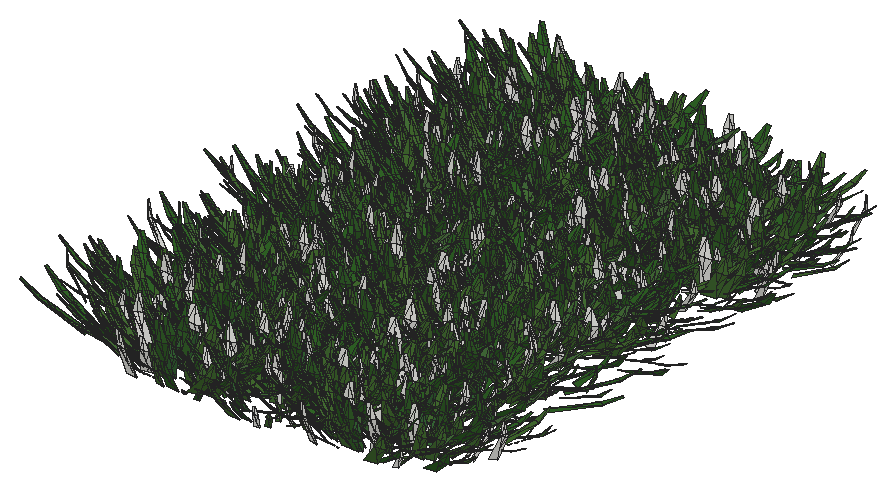
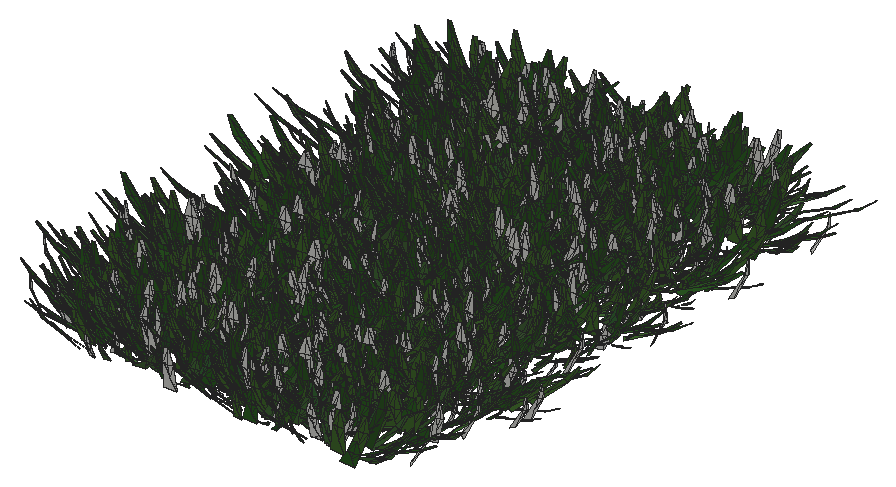
# SketchUp Ruby script. Lengths in inches.
U = 1.inch
M = Sketchup.active_model
def pt(a) = Geom::Point3d.new(a.map { |v| v * U })
def face(e, loops, mat)
  f = e.add_face(loops[0].map { |a| pt(a) })
  loops[1..].each { |l| e.add_face(l.map { |a| pt(a) }).erase! }
  f.material = f.back_material = mat if mat
  f
end
# faces: each face lists its corners as indices into pts; further lists are holes
def faces(e, pts, list, mat = nil) = list.each { |f| face(e, (f[0].is_a?(Array) ? f : [f]).map { |l| l.map { |i| pts[i] } }, mat) }
# xy, xz, yz: faces in a plane at the given z, y or x. An outline is a flat list of corners, or four numbers for a rectangle; further outlines are holes
def ring(l) = l.size == 4 ? [[l[0], l[1]], [l[2], l[1]], [l[2], l[3]], [l[0], l[3]]] : l.each_slice(2).to_a
def flat(e, list, mat, &to3) = list.each { |f| face(e, (f[0].is_a?(Array) ? f : [f]).map { |l| ring(l).map { |u, v| to3.(u, v) } }, mat) }
def xy(e, z, list, mat = nil) = flat(e, list, mat) { |x, y| [x, y, z] }
def xz(e, y, list, mat = nil) = flat(e, list, mat) { |x, z| [x, y, z] }
def yz(e, x, list, mat = nil) = flat(e, list, mat) { |y, z| [x, y, z] }
def lines(e, pts, list) = list.each { |a, b| e.add_line(pt(pts[a]), pt(pts[b])) }
# prism: a flat outline (further loops are holes) pulled along v
def prism(e, loops, v, mat = nil)
  f = face(e, loops, mat); d = Geom::Vector3d.new(v.map { |x| x * U })
  f.pushpull(f.normal.samedirection?(d) ? d.length : -d.length)
end
def box(e, o, s, mat = nil) = prism(e, [[o, [o[0] + s[0], o[1], o[2]], [o[0] + s[0], o[1] + s[1], o[2]], [o[0], o[1] + s[1], o[2]]]], [0, 0, s[2]], mat)
def at(x, y, z, deg = 0) = Geom::Transformation.translation(pt([x, y, z])) * Geom::Transformation.rotation(ORIGIN, Z_AXIS, deg.degrees)
def axes(o, x, y, z) = Geom::Transformation.new([*x, 0, *y, 0, *z, 0, *pt(o).to_a, 1])
def part(name) = M.definitions.add(name)
# library, detail: a bought-in or finely detailed component or shape, given as its bounding box
def library(name, o, s) = part(name).tap { |d| box(d.entities, o, s) }
def detail(e, o, s) = box(e.add_group.entities, o, s)
def put(e, d, t, mat = nil) = e.add_instance(d, t).tap { |i| i.material = mat if mat }
def group(e, t, mat = nil) = e.add_group.tap { |g| g.transformation = t; g.material = mat if mat }.entities
root = M.entities
M.materials.add("Material82").color = [68, 110, 58]
M.materials.add("Material83").color = [48, 90, 38]
M.materials.add("Material84").color = [68, 110, 48]
M.materials.add("Material85").color = [48, 90, 48]
M.materials.add("Material86").color = [58, 110, 58]
M.materials.add("Material87").color = [58, 90, 38]
M.materials.add("Material88").color = [68, 100, 58]
M.materials.add("Material89").color = [48, 100, 38]
c1 = part("grass00")
p = [[-0.6875,0.15,0],[-0.56,0.08,5.52],[-0.04,0.03,2.76],[0.48,-0.02,0],[0.35,-0.02,5.52],[-0.1,-0.14,5.52],
  [-0.12,0.65,8.37],[-0.42,0.65,8.37]]
faces(c1.entities,p,[[0,1,2,3],[3,2,4],[1,5,2],[5,4,2],[1,6,5],[4,5,6],[7,6,1]])
c2 = part("Group16\#1")
put(c2.entities,c1,axes([1.44,-0.61,-0.01],[0.05352,0.12609,0],[-0.10704,0.04543,0.07239],[0.06664,-0.02828,0.11628]),"Material85")
put(c2.entities,c1,axes([0.76,-0.15,-0.01],[0.04676,0.24062,0],[-0.23162,0.04501,0.06642],[0.0652,-0.01267,0.23595]),"Material82")
put(c2.entities,c1,axes([0.79,0.01,-0.01],[-0.00606,0.34651,0],[-0.34381,-0.00602,0.0432],[0.04319,0.00076,0.34386]))
put(c2.entities,c1,axes([1,0.23,-0.01],[-0.07192,0.31144,0],[-0.28722,-0.06632,0.1236],[0.12043,0.02781,0.29478]),"Material84")
put(c2.entities,c1,axes([1.66,0.77,-0.01],[-0.13828,0.29651,0],[-0.21551,-0.1005,0.22471],[0.20365,0.09498,0.23779]),"Material89")
put(c2.entities,c1,axes([0.6875,0.52,-0.01],[-0.18126,0.24051,0],[-0.22746,-0.17142,0.09788],[0.07817,0.05891,0.28481]),"Material84")
put(c2.entities,c1,axes([0.68,0.78,-0.01],[-0.215,0.18688,0],[-0.12385,-0.14248,0.21334],[0.13995,0.16101,0.18878]),"Material82")
put(c2.entities,c1,axes([0.56,1,-0.01],[-0.13756,0.07624,0],[-0.06159,-0.11112,0.0927],[0.04494,0.08108,0.12705]),"Material84")
put(c2.entities,c1,axes([0.2,0.64,-0.01],[-0.23729,0.07254,0],[-0.05711,-0.18681,0.153],[0.04473,0.14632,0.19535]),"Material89")
put(c2.entities,c1,axes([0.0625,0.72,-0.01],[-0.28874,0.02525,0],[-0.02179,-0.24916,0.14647],[0.01276,0.14591,0.25012]),"Material82")
put(c2.entities,c1,axes([-0.08,0.62,-0.01],[-0.34089,-0.04187,0],[0.03255,-0.26504,0.216],[-0.02633,0.21439,0.26703]),"Material89")
put(c2.entities,c1,axes([-0.34,0.98,-0.01],[-0.14314,-0.0493,0],[0.04397,-0.12769,0.06843],[-0.02228,0.0647,0.13505]),"Material89")
put(c2.entities,c1,axes([-0.87,1.45,-0.01],[-0.23488,-0.14114,0],[0.13761,-0.22901,0.06087],[-0.03135,0.05217,0.26717]))
put(c2.entities,c1,axes([-0.72,0.77,-0.01],[-0.14208,-0.13251,0],[0.07209,-0.0773,0.16301],[-0.11118,0.11922,0.1057]),"Material89")
put(c2.entities,c1,axes([-0.62,0.43,-0.01],[-0.14845,-0.21203,0],[0.18654,-0.13061,0.12304],[-0.10079,0.07057,0.22772]),"Material82")
put(c2.entities,c1,axes([-0.68,0.29,-0.01],[-0.13639,-0.32136,0],[0.31723,-0.13464,0.05579],[-0.05136,0.0218,0.34462]),"Material83")
put(c2.entities,c1,axes([-0.64,0.125,-0.01],[-0.0458,-0.23569,0],[0.22124,-0.043,0.08276],[-0.08124,0.01579,0.22538]),"Material86")
put(c2.entities,c1,axes([-1.6,-0.03,-0.01],[0.00576,-0.32897,0],[0.27526,0.00482,0.18018],[-0.18015,-0.00315,0.2753]),"Material84")
put(c2.entities,c1,axes([-1.36,-0.31,-0.01],[0.05718,-0.24765,0],[0.18172,0.04196,0.17267],[-0.16825,-0.03885,0.1865]),"Material89")
put(c2.entities,c1,axes([-1.54,-0.72,-0.01],[0.06537,-0.14017,0],[0.13555,0.06321,0.03939],[-0.0357,-0.01665,0.14956]))
put(c2.entities,c1,axes([-1.19,-0.9,-0.01],[0.09597,-0.12735,0],[0.11214,0.08451,0.07557],[-0.06035,-0.04548,0.14042]),"Material88")
put(c2.entities,c1,axes([-0.47,-0.54,-0.01],[0.11588,-0.10072,0],[0.0618,0.0711,0.12124],[-0.07953,-0.0915,0.0942]))
put(c2.entities,c1,axes([-0.47,-0.84,-0.01],[0.11927,-0.0661,0],[0.06603,0.11913,0.00646],[-0.00313,-0.00565,0.13621]),"Material84")
put(c2.entities,c1,axes([-0.38,-1.24,-0.01],[0.28037,-0.08571,0],[0.0618,0.20215,0.20315],[-0.05939,-0.19428,0.21139]),"Material88")
put(c2.entities,c1,axes([-0.06,-0.66,-0.01],[0.22719,-0.01987,0],[0.01247,0.14255,0.17758],[-0.01547,-0.17691,0.1431]),"Material87")
put(c2.entities,c1,axes([0.11,-0.89,-0.01],[0.14882,0.01828,0],[-0.01058,0.08611,0.12229],[0.01491,-0.12138,0.08676]),"Material85")
put(c2.entities,c1,axes([0.25,-0.72,-0.01],[0.20481,0.07053,0],[-0.06206,0.18022,0.10291],[0.03351,-0.0973,0.1906]),"Material85")
put(c2.entities,c1,axes([0.85,-1.42,-0.01],[0.16481,0.09904,0],[-0.09472,0.15762,0.05616],[0.02893,-0.04814,0.18389]),"Material84")
put(c2.entities,c1,axes([1.01,-1.09,-0.01],[0.21858,0.20385,0],[-0.17495,0.1876,0.15339],[0.10462,-0.11218,0.25652]),"Material89")
put(c2.entities,c1,axes([1.01,-0.71,-0.01],[0.08733,0.12473,0],[-0.06445,0.04512,0.13037],[0.1068,-0.07477,0.07867]),"Material85")
c3 = part("Group15\#1")
put(c3.entities,c2,at(0,0,0))
c4 = part("3darcstudiotree_grass00\#1")
put(c4.entities,c3,at(0,0,0))
put(root,c4,axes([1794.49,955.9,-29.74],[2.02269,1.40625,0],[-2.88305,0.64496,-0.03898],[-0.27125,0.06068,1.98748]))
put(root,c4,axes([1794.85,983.84,-29.74],[2.29641,1.07421,0],[-2.57105,0.85483,-0.04117],[-0.19383,0.06444,1.55213]))
put(root,c4,axes([1794.83,946.6,-29.74],[0.20899,1.64265,0],[-4.27343,0.08456,-0.03261],[-0.1888,0.00374,1.85888]))
put(root,c4,axes([1794.68,966.71,-29.74],[1.08869,1.44245,0],[-3.40274,0.39943,-0.00785],[-0.05372,0.00631,1.89978]))
put(root,c4,axes([1794.9,981.94,-29.74],[2.7006,1.1614,0],[-2.43909,0.8821,-0.03804],[-0.19893,0.07194,1.7602]))
put(root,c4,axes([1797.5625,973.19,-29.74],[-2.45174,-1.03973,0],[2.50397,-0.91832,-0.03633],[0.18002,-0.06602,1.73438]))
put(root,c4,axes([1797.66,970.78,-29.74],[-1.7758,-1.16797,0],[3.11451,-0.73649,-0.04451],[0.21848,-0.05166,1.55797]))
put(root,c4,axes([1798.16,960.11,-29.74],[-4.0045,-0.70324,0],[1.53901,-1.36302,-0.04343],[0.08424,-0.0746,1.35201]))
put(root,c4,axes([1797.9,953.62,-29.74],[-0.8562,-1.46222,0],[3.2715,-0.29793,-0.0292],[0.1741,-0.01586,1.53984]))
put(root,c4,axes([1797.63,961.45,-29.74],[2.12424,-1.58648,0],[2.98317,0.62124,-0.03491],[0.20173,0.04201,1.65255]))
put(root,c4,axes([1798.36,942.04,-29.74],[-3.45178,0.2701,0],[-0.90786,-1.80446,-0.05548],[-0.0508,-0.10098,1.6451]))
put(root,c4,axes([1799.49,982.04,-29.74],[-3.12186,-1.16816,0],[2.84193,-1.18123,-0.00166],[0.00643,-0.00267,1.74215]))
put(root,c4,axes([1797.65,988.83,-29.74],[3.25093,0.54248,0],[-1.41803,1.32165,-0.02719],[-0.07494,0.06985,1.929]))
put(root,c4,axes([1797.67,989.51,-29.74],[-0.25702,1.50589,0],[-4.4334,-0.11768,-0.01753],[-0.09867,-0.00262,1.87889]))
put(root,c4,axes([1797.58,967.875,-29.74],[3.97101,0.68213,0],[-1.55734,1.41002,-0.04191],[-0.07595,0.06876,1.32656]))
put(root,c4,axes([1798.15,995.21,-29.74],[0.4621,1.41992,0],[-4.03416,0.20419,-0.0516],[-0.33532,0.01697,1.99718]))
put(root,c4,axes([1797.97,977.52,-29.74],[4.12561,0.29265,0],[-0.72369,1.58676,-0.03729],[-0.0346,0.07587,1.60628]))
put(root,c4,axes([1799.72,950.6,-29.74],[-3.96689,-0.26306,0],[0.64548,-1.51387,-0.0114],[0.01279,-0.03,1.97478]))
put(root,c4,axes([1798.23,974.62,-29.74],[2.01819,1.66422,0],[-3.45385,0.65143,-0.02212],[-0.1358,0.02561,1.95299]))
put(root,c4,axes([1798.51,958.22,-29.74],[-0.26486,1.49696,0],[-3.89065,-0.10706,-0.02357],[-0.1242,-0.00342,1.54387]))
put(root,c4,axes([1798.52,948.51,-29.74],[4.24203,-0.02956,0],[0.08072,1.80172,-0.02875],[0.00231,0.05162,1.55972]))
put(root,c4,axes([1798.66,983.97,-29.74],[2.46344,0.86677,0],[-2.31784,1.02455,-0.00625],[-0.02756,0.01218,1.72796]))
put(root,c4,axes([1800.12,965.53,-29.74],[-3.7951,0.9119,0],[-2.12877,-1.37789,-0.05764],[-0.17628,-0.1141,1.8024]))
put(root,c4,axes([1800.5,944.45,-29.74],[1.13972,-1.41461,0],[4.50389,0.56436,-0.03698],[0.18209,0.02282,1.82987]))
put(root,c4,axes([1801.0625,954.77,-29.74],[-2.49551,-1.26471,0],[2.8619,-0.87828,-0.01663],[0.09126,-0.02801,1.89037]))
put(root,c4,axes([1800.7,940.35,-29.74],[-2.98133,1.10226,0],[-2.6348,-1.10837,-0.04557],[-0.21161,-0.08902,1.96028]))
put(root,c4,axes([1800.3125,978.84,-29.74],[-2.13819,1.22316,0],[-3.167,-0.86103,-0.02321],[-0.1127,-0.03064,1.70026]))
put(root,c4,axes([1800.97,947.39,-29.74],[-3.3677,0.38425,0],[-1.22656,-1.67195,-0.00573],[-0.0077,-0.0105,1.59925]))
put(root,c4,axes([1800.92,986.4,-29.74],[2.12809,-1.0558,0],[3.61722,1.13396,-0.06111],[0.24603,0.07713,1.78135]))
put(root,c4,axes([1801.03,993.1,-29.74],[3.47556,-0.63984,0],[1.81232,1.53108,-0.02938],[0.06383,0.05392,1.64954]))
put(root,c4,axes([1800.85,964.29,-29.74],[4.6709,-0.11713,0],[0.23839,1.47848,-0.03177],[0.01367,0.08477,1.90853]))
put(root,c4,axes([1803.0625,971.1,-29.74],[-3.65792,-0.8597,0],[1.995,-1.32021,-0.01663],[0.05672,-0.03754,1.94585]))
put(root,c4,axes([1803.21,940.4,-29.74],[3.22982,-1.36398,0],[2.52221,0.92889,-0.01281],[0.05669,0.02088,1.56626]))
put(root,c4,axes([1804.68,966.21,-29.74],[-1.61628,-1.19973,0],[3.67441,-0.7699,-0.00698],[0.03732,-0.00782,1.8873]))
put(root,c4,axes([1804.32,944.1875,-29.74],[1.53079,-1.5017,0],[4.19952,0.6658,-0.01772],[0.08663,0.01374,1.7874]))
put(root,c4,axes([1804.85,953.47,-29.74],[-3.12873,-1.31633,0],[2.88309,-1.0658,-0.03051],[0.12402,-0.04585,1.65027]))
put(root,c4,axes([1804.24,991.84,-29.74],[2.10607,-1.53284,0],[3.55653,0.76,-0.00988],[0.05409,0.01156,1.88737]))
put(root,c4,axes([1803.2,959.43,-29.74],[4.72899,0.01401,0],[-0.03317,1.74196,-0.012],[-0.00046,0.02441,1.70791]))
put(root,c4,axes([1803.95,942.24,-29.74],[3.14565,-0.76847,0],[1.85222,1.17921,-0.00486],[0.01386,0.00882,1.42853]))
put(root,c4,axes([1803.34,961.83,-29.74],[1.47307,1.52241,0],[-3.55442,0.5349,-0.03212],[-0.18221,0.02742,1.73128]))
put(root,c4,axes([1803.71,948.7,-29.74],[3.86384,0.07818,0],[-0.23972,1.84255,-0.05168],[-0.01275,0.09801,1.68853]))
put(root,c4,axes([1803.54,955.48,-29.74],[0.17144,1.84869,0],[-4.60552,0.06643,-0.0182],[-0.07619,0.0011,1.44668]))
put(root,c4,axes([1803.7,974.37,-29.74],[0.6087,1.43701,0],[-3.38203,0.22281,-0.00028],[-0.00164,0.00011,1.50491]))
put(root,c4,axes([1804.01,990.32,-29.74],[-0.11554,1.45354,0],[-4.02615,-0.04978,-0.04067],[-0.20655,-0.00255,1.53414]))
put(root,c4,axes([1804.83,981.89,-29.74],[-3.14808,1.22755,0],[-2.57668,-1.02773,-0.03762],[-0.14164,-0.05649,1.47105]))
put(root,c4,axes([1803.68,986.65,-29.74],[0.48824,1.58889,0],[-4.56618,0.21822,-0.01569],[-0.06712,0.00321,1.48562]))
put(root,c4,axes([1805.84,977.55,-29.74],[-3.3453,-1.30601,0],[3.28392,-1.30825,-0.03717],[0.14464,-0.05762,1.93537]))
put(root,c4,axes([1805.64,972.4,-29.74],[-4.03093,-0.26709,0],[0.61626,-1.44652,-0.01654],[0.01865,-0.04378,1.89711]))
put(root,c4,axes([1806.03,978.98,-29.74],[-1.63649,-1.29377,0],[3.38922,-0.66676,-0.00448],[0.02699,-0.00531,1.90991]))
put(root,c4,axes([1805.21,958.33,-29.74],[-3.19374,0.7238,0],[-2.32014,-1.59223,-0.04948],[-0.1132,-0.07768,1.60238]))
put(root,c4,axes([1804.66,984.03,-29.74],[0.67214,1.30105,0],[-3.68417,0.29602,-0.04728],[-0.27019,0.02171,1.64346]))
put(root,c4,axes([1804.99,968.28,-29.74],[3.23921,0.6316,0],[-1.61427,1.28761,-0.03066],[-0.08714,0.06951,1.75054]))
put(root,c4,axes([1806.09,947.34,-29.74],[0.38628,-1.42854,0],[3.50239,0.14729,-0.04937],[0.32013,0.01346,1.72169]))
put(root,c4,axes([1806.32,963.77,-29.74],[-1.61807,1.52118,0],[-3.6405,-0.60227,-0.04701],[-0.26943,-0.04457,1.83905]))
put(root,c4,axes([1806.52,951.08,-29.74],[0.41177,1.61489,0],[-3.5087,0.13914,-0.04963],[-0.27633,0.01096,1.47912]))
put(root,c4,axes([1805.89,994.14,-29.74],[3.03872,1.12896,0],[-3.11924,1.30579,-0.01047],[-0.04051,0.01696,1.92288]))
put(root,c4,axes([1806.92,987.59,-29.74],[3.86781,0.52244,0],[-1.13731,1.30954,-0.02009],[-0.0432,0.04974,1.7458]))
put(root,c4,axes([1808.63,986.48,-29.74],[-4.0386,-0.4374,0],[0.94795,-1.36128,-0.02848],[0.0516,-0.0741,1.83531]))
put(root,c4,axes([1808.37,992.54,-29.74],[-0.39879,-1.78911,0],[3.98788,-0.13825,-0.04765],[0.27848,-0.00965,1.76037]))
put(root,c4,axes([1808.59,995.03,-29.74],[-3.75498,0.92244,0],[-1.75834,-1.11323,-0.01072],[-0.04199,-0.02659,1.84718]))
put(root,c4,axes([1809.13,955.28,-29.74],[-3.9685,0.8355,0],[-2.02289,-1.49439,-0.03463],[-0.09424,-0.06962,1.86049]))
put(root,c4,axes([1808.72,962.1875,-29.74],[-1.70053,1.52985,0],[-3.13018,-0.54115,-0.01229],[-0.08699,-0.01504,1.9803]))
put(root,c4,axes([1810.13,983.63,-29.74],[-3.28059,-1.08182,0],[2.91353,-1.37413,-0.04137],[0.10673,-0.05034,1.36909]))
put(root,c4,axes([1809.65,975.17,-29.74],[3.17929,-0.7211,0],[2.23361,1.53163,-0.03788],[0.07878,0.05402,1.40078]))
put(root,c4,axes([1809.07,972.49,-29.74],[4.05026,0.33604,0],[-0.7921,1.48485,-0.04482],[-0.0484,0.09073,1.51278]))
put(root,c4,axes([1810.84,987.75,-29.74],[-2.84597,-0.98358,0],[2.28129,-1.02662,-0.01406],[0.06335,-0.02851,1.77353]))
put(root,c4,axes([1810.01,981.77,-29.74],[3.81863,-0.53813,0],[1.40932,1.55539,-0.0155],[0.0332,0.03664,1.9985]))
put(root,c4,axes([1811.33,949.61,-29.74],[-2.42754,-1.16571,0],[2.71881,-0.88058,-0.021],[0.08634,-0.02796,1.40308]))
put(root,c4,axes([1811.26,956.96,-29.74],[-1.73285,-1.40976,0],[3.20349,-0.61242,-0.03263],[0.20579,-0.03934,1.87]))
put(root,c4,axes([1810.17,979.68,-29.74],[3.58142,-0.447,0],[1.06233,1.32378,-0.04021],[0.07095,0.08841,1.5432]))
put(root,c4,axes([1811.43,953.95,-29.74],[-4.30499,0.20084,0],[-0.50439,-1.68151,-0.02284],[-0.01208,-0.04026,1.44864]))
put(root,c4,axes([1810.89,946.27,-29.74],[-2.18902,1.07825,0],[-2.9207,-0.92221,-0.02462],[-0.13408,-0.04234,1.95656]))
put(root,c4,axes([1810.3125,942.99,-29.74],[2.94971,1.39882,0],[-3.26889,1.07209,-0.02991],[-0.14108,0.04627,1.95467]))
put(root,c4,axes([1812.17,964.38,-29.74],[0.02605,-1.38879,0],[4.64619,0.01356,-0.04606],[0.23946,0.0007,1.81052]))
put(root,c4,axes([1810.59,966.1,-29.74],[3.34775,0.73741,0],[-1.81639,1.28251,-0.02091],[-0.0568,0.0401,1.55496]))
put(root,c4,axes([1810.5,977.25,-29.74],[4.2068,0.84458,0],[-2.08885,1.6182,-0.01612],[-0.03432,0.02659,1.61949]))
put(root,c4,axes([1811.95,969.12,-29.74],[-3.54698,0.73807,0],[-1.81276,-1.35492,-0.01893],[-0.04162,-0.0311,1.37131]))
put(root,c4,axes([1811.97,944.96,-29.74],[-3.36311,0.85521,0],[-1.93534,-1.1837,-0.01497],[-0.0443,-0.0271,1.4615]))
put(root,c4,axes([1811.34,940.16,-29.74],[0.45304,1.69594,0],[-3.37186,0.14009,-0.01763],[-0.11097,0.00461,1.60818]))
put(root,c4,axes([1811.57,970.46,-29.74],[2.84839,1.04367,0],[-2.27167,0.96426,-0.03885],[-0.20657,0.08768,1.95422]))
put(root,c4,axes([1812.09,989.98,-29.74],[3.6343,-0.40762,0],[1.19135,1.65202,-0.03545],[0.05267,0.07304,1.77295]))
put(root,c4,axes([1811.8,959.63,-29.74],[0.87217,1.79185,0],[-4.36686,0.33058,-0.02457],[-0.1156,0.00875,1.59681]))
put(root,c4,axes([1812.38,950.48,-29.74],[3.8213,1.10557,0],[-2.37941,1.27911,-0.00415],[-0.01079,0.0058,1.32509]))
put(root,c4,axes([1813.92,955.88,-29.74],[1.36885,-1.43158,0],[3.98655,0.59286,-0.04892],[0.27754,0.04127,1.93615]))
put(root,c4,axes([1814.58,975.04,-29.74],[-3.05635,-0.6343,0],[1.70161,-1.2752,-0.01604],[0.05188,-0.03888,1.9024]))
put(root,c4,axes([1814.73,983.79,-29.74],[-0.79946,-1.53657,0],[4.27905,-0.34626,-0.03341],[0.18605,-0.01506,1.86102]))
put(root,c4,axes([1814.37,953.25,-29.74],[1.53865,-1.45346,0],[4.25105,0.69992,-0.03949],[0.18935,0.03118,1.7941]))
put(root,c4,axes([1815.02,967.02,-29.74],[-2.53143,-1.15701,0],[3.22557,-1.09761,-0.03179],[0.10043,-0.03417,1.33245]))
put(root,c4,axes([1815.53,978.59,-29.74],[0.41929,-1.46273,0],[4.6699,0.2082,-0.01256],[0.06761,0.00301,1.90836]))
put(root,c4,axes([1814,945.1,-29.74],[3.57437,0.42668,0],[-1.04232,1.35805,-0.0422],[-0.08519,0.111,1.87907]))
put(root,c4,axes([1814.42,967.68,-29.74],[4.54472,-0.07638,0],[0.17813,1.64846,-0.04096],[0.00957,0.08859,1.72127]))
put(root,c4,axes([1816.21,959.96,-29.74],[-1.16799,-1.2811,0],[3.57696,-0.50721,-0.0171],[0.1013,-0.01436,1.79343]))
put(root,c4,axes([1815.84,992.61,-29.74],[-4.37429,0.70017,0],[-1.56113,-1.51689,-0.01879],[-0.03338,-0.03243,1.46955]))
put(root,c4,axes([1816.16,951.32,-29.74],[-3.24054,-0.28468,0],[0.77392,-1.37016,-0.02543],[0.03342,-0.05916,1.61262]))
put(root,c4,axes([1815.59,981.88,-29.74],[-2.88569,0.96312,0],[-2.81786,-1.31311,-0.05904],[-0.17262,-0.08044,1.47981]))
put(root,c4,axes([1816.37,948.71,-29.74],[1.16933,-1.48396,0],[3.883,0.47588,-0.02169],[0.1048,0.01284,1.54236]))
put(root,c4,axes([1816.83,945.8125,-29.74],[-0.65586,-1.46962,0],[4.60144,-0.31938,-0.05842],[0.32577,-0.02261,1.98292]))
put(root,c4,axes([1816.02,971.44,-29.74],[3.94842,-0.68884,0],[1.45256,1.29494,-0.00969],[0.01982,0.01767,1.36001]))
put(root,c4,axes([1817.36,963.67,-29.74],[-3.73914,-0.79189,0],[1.71097,-1.25649,-0.0264],[0.09118,-0.06696,1.979]))
put(root,c4,axes([1817.21,989.64,-29.74],[-3.92506,-0.07313,0],[0.21494,-1.79423,-0.03065],[0.00834,-0.06965,1.9691]))
put(root,c4,axes([1815.6,973.37,-29.74],[4.38423,0.4309,0],[-1.14012,1.80418,-0.03274],[-0.03634,0.0575,1.62193]))
put(root,c4,axes([1817.51,957.5,-29.74],[-3.57377,-0.68668,0],[1.88387,-1.52489,-0.02869],[0.074,-0.0599,1.89824]))
put(root,c4,axes([1816.01,961.16,-29.74],[4.39904,-0.03006,0],[0.06093,1.38656,-0.04649],[0.00481,0.10943,1.57333]))
put(root,c4,axes([1816.76,994.33,-29.74],[3.99314,-0.58395,0],[1.40862,1.49812,-0.01564],[0.03379,0.03593,1.88746]))
put(root,c4,axes([1816.87,987.28,-29.74],[-1.29956,1.24249,0],[-3.63161,-0.59077,-0.01866],[-0.09119,-0.01483,1.55626]))
put(root,c4,axes([1817.47,976.875,-29.74],[4.62104,-0.01455,0],[0.03483,1.71996,-0.00522],[0.00018,0.00901,1.42947]))
put(root,c4,axes([1817.66,985.5,-29.74],[1.74244,1.18271,0],[-3.27168,0.74965,-0.03711],[-0.19162,0.04391,1.69359]))
put(root,c4,axes([1817.51,941.69,-29.74],[2.60331,1.05125,0],[-2.58261,0.9947,-0.01838],[-0.08057,0.03103,1.65818]))
put(root,c4,axes([1819.64,962.15,-29.74],[-4.17671,-0.8199,0],[2.05439,-1.62767,-0.0574],[0.10467,-0.08292,1.41402]))
put(root,c4,axes([1819.96,992.11,-29.74],[-3.98486,0.06108,0],[-0.1339,-1.35868,-0.04521],[-0.01298,-0.1317,1.91035]))
put(root,c4,axes([1820.4,981.68,-29.74],[-3.51388,-0.90483,0],[2.14031,-1.29273,-0.0556],[0.17294,-0.10445,1.66946]))
put(root,c4,axes([1819.45,968.93,-29.74],[-2.56609,1.18757,0],[-3.37526,-1.13431,-0.01912],[-0.05922,-0.0199,1.35238]))
put(root,c4,axes([1820.64,950.59,-29.74],[-3.1974,-0.52057,0],[1.31873,-1.25975,-0.01181],[0.03016,-0.02882,1.73426]))
put(root,c4,axes([1820.49,959.85,-29.74],[-0.51556,-1.46046,0],[3.95081,-0.21691,-0.04493],[0.28513,-0.01565,1.91565]))
put(root,c4,axes([1820.58,989.8125,-29.74],[0.81424,-1.34129,0],[3.64589,0.34423,-0.00366],[0.01919,0.00181,1.51551]))
put(root,c4,axes([1821.11,949.61,-29.74],[0.21445,-1.64927,0],[3.6182,0.07317,-0.01161],[0.06174,0.00125,1.44612]))
put(root,c4,axes([1821.73,975.71,-29.74],[-3.21256,-1.12789,0],[2.70503,-1.19832,-0.03256],[0.11538,-0.05111,1.62483]))
put(root,c4,axes([1821.81,979.87,-29.74],[-3.59955,0.15303,0],[-0.4164,-1.52331,-0.01956],[-0.01422,-0.05201,1.97453]))
put(root,c4,axes([1820.55,942.38,-29.74],[-0.10583,1.54224,0],[-3.7996,-0.04055,-0.00627],[-0.03571,-0.00038,1.62459]))
put(root,c4,axes([1822.33,994.14,-29.74],[-2.41013,-1.27132,0],[2.91819,-0.86042,-0.02089],[0.0972,-0.02866,1.58683]))
put(root,c4,axes([1821.7,955.47,-29.74],[-3.10318,1.24143,0],[-2.60712,-1.01358,-0.05097],[-0.2393,-0.09303,1.80901]))
put(root,c4,axes([1821.32,940.45,-29.74],[-1.86859,1.14232,0],[-3.14905,-0.80116,-0.00439],[-0.02189,-0.00557,1.66469]))
put(root,c4,axes([1821.3,988.09,-29.74],[-1.19351,1.65501,0],[-3.6228,-0.40633,-0.01558],[-0.10093,-0.01132,1.90128]))
put(root,c4,axes([1820.9,965.58,-29.74],[3.31436,0.96989,0],[-2.30719,1.22623,-0.02502],[-0.09786,0.05201,1.90511]))
put(root,c4,axes([1822.94,985.85,-29.74],[-1.03972,-1.40109,0],[4.3795,-0.50546,-0.04795],[0.2061,-0.02379,1.53186]))
put(root,c4,axes([1821.5,946.2,-29.74],[-0.80891,1.58211,0],[-4.50454,-0.3582,-0.03197],[-0.1625,-0.01292,1.78572]))
put(root,c4,axes([1822.81,944.49,-29.74],[-3.61232,0.8121,0],[-2.24589,-1.55373,-0.01918],[-0.05035,-0.03483,1.80194]))
put(root,c4,axes([1822.85,963.6,-29.74],[1.76506,-1.25364,0],[3.37171,0.73833,-0.03203],[0.17156,0.03757,1.771]))
put(root,c4,axes([1822.74,984.46,-29.74],[-2.8527,1.28628,0],[-3.36111,-1.15935,-0.03347],[-0.14409,-0.0497,1.91416]))
put(root,c4,axes([1822.18,956.76,-29.74],[4.4529,0.04613,0],[-0.09862,1.48061,-0.04419],[-0.00818,0.12282,1.98467]))
put(root,c4,axes([1823.53,977.03,-29.74],[-4.01452,0.69277,0],[-1.67449,-1.50916,-0.02625],[-0.04914,-0.04429,1.46233]))
put(root,c4,axes([1822.74,970.14,-29.74],[-0.38971,1.40175,0],[-3.70548,-0.16023,-0.02456],[-0.14917,-0.00645,1.70727]))
put(root,c4,axes([1822.7,953.01,-29.74],[4.64374,0.18316,0],[-0.43015,1.69615,-0.02551],[-0.01161,0.04577,1.48132]))
put(root,c4,axes([1823.28,972.26,-29.74],[3.33641,-0.4539,0],[1.10224,1.26009,-0.03311],[0.06709,0.0767,1.57439]))
put(root,c4,axes([1825.4375,984.49,-29.74],[-4.08837,-0.48406,0],[1.24556,-1.63618,-0.01736],[0.02056,-0.027,1.33702]))
put(root,c4,axes([1825.26,965.96,-29.74],[1.677,-1.55355,0],[4.28787,0.71988,-0.03539],[0.14144,0.02375,1.51703]))
put(root,c4,axes([1825.71,981.15,-29.74],[-2.71685,-1.17622,0],[2.71806,-0.97644,-0.02128],[0.11147,-0.04005,1.95268]))
put(root,c4,axes([1825.96,945.82,-29.74],[-3.01218,-1.1682,0],[2.32929,-0.93411,-0.00764],[0.03903,-0.01565,1.81511]))
put(root,c4,axes([1826,992.61,-29.74],[0.25601,-1.60576,0],[3.7655,0.09337,-0.00515],[0.03185,0.00079,1.75106]))
put(root,c4,axes([1825.01,971.13,-29.74],[-1.88352,1.24088,0],[-3.53635,-0.83485,-0.03562],[-0.13641,-0.0322,1.37892]))
put(root,c4,axes([1825.73,943.02,-29.74],[0.35251,-1.39793,0],[3.51175,0.13773,-0.03727],[0.24286,0.00952,1.73202]))
put(root,c4,axes([1826,948.76,-29.74],[-3.43821,0.20499,0],[-0.69374,-1.80975,-0.03474],[-0.02131,-0.0556,1.42794]))
put(root,c4,axes([1825.06,957.77,-29.74],[-0.07716,1.61232,0],[-4.08051,-0.03037,-0.05443],[-0.27918,-0.00208,1.56933]))
put(root,c4,axes([1826.6,979.31,-29.74],[1.28288,-1.22527,0],[4.05082,0.65965,-0.04448],[0.2416,0.03934,1.93016]))
put(root,c4,axes([1826.875,987.7,-29.74],[-0.2981,-1.54731,0],[4.18924,-0.12553,-0.05563],[0.33136,-0.00993,1.88098]))
